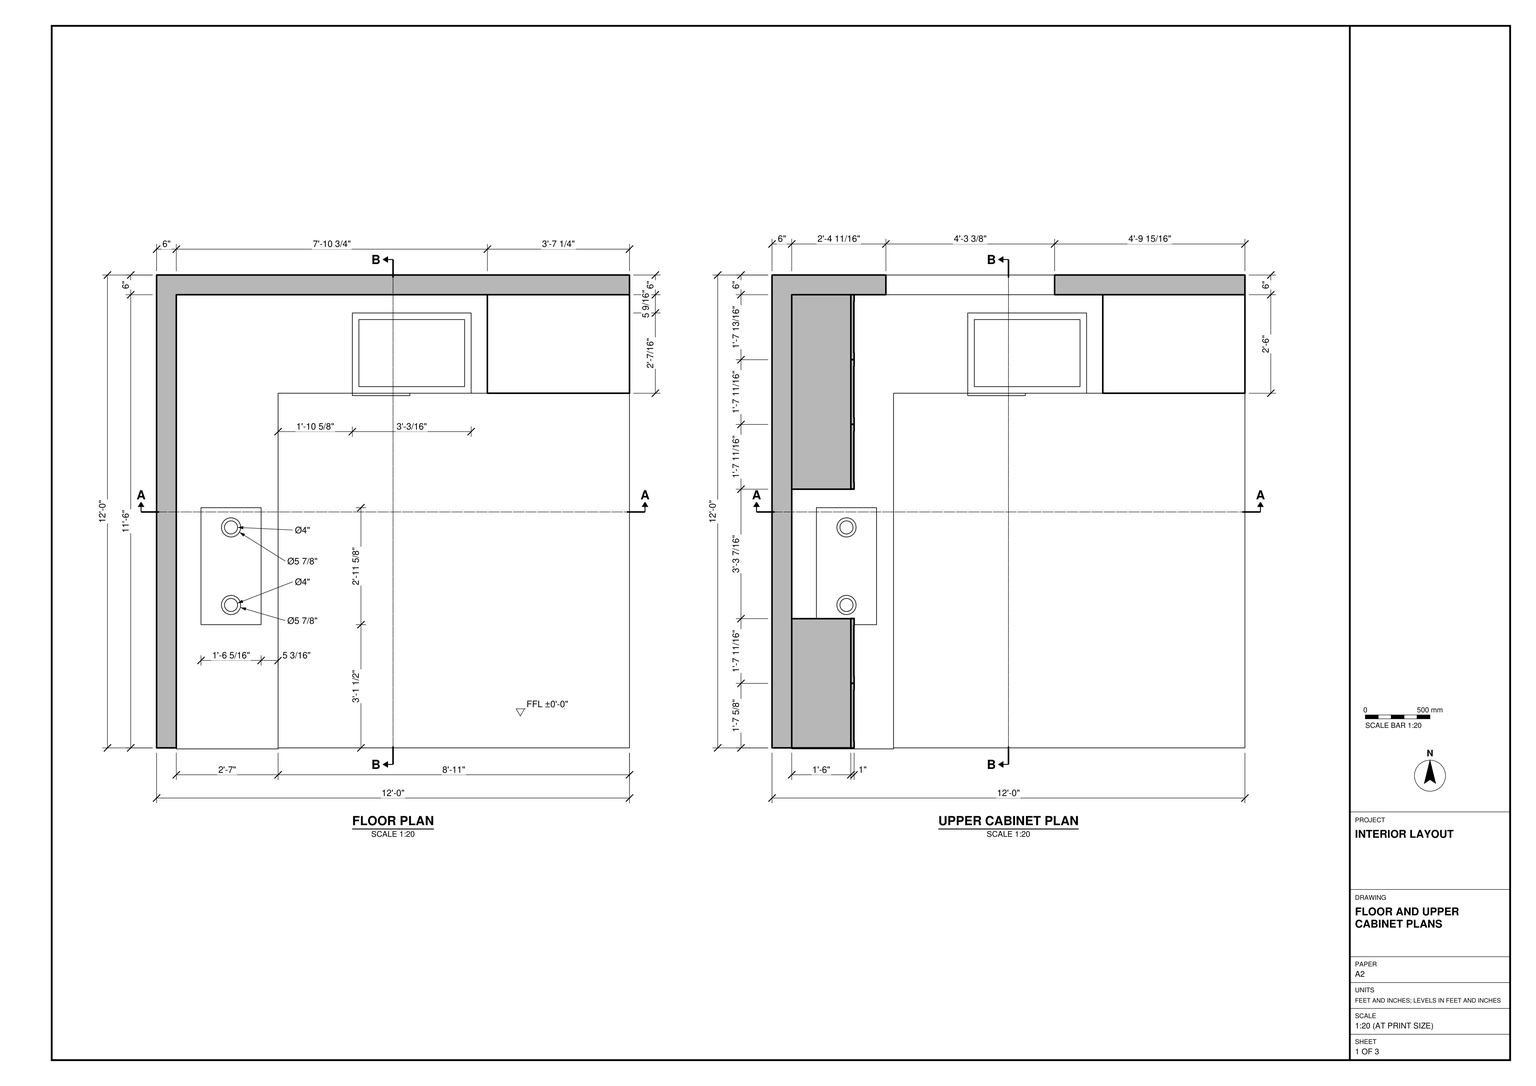
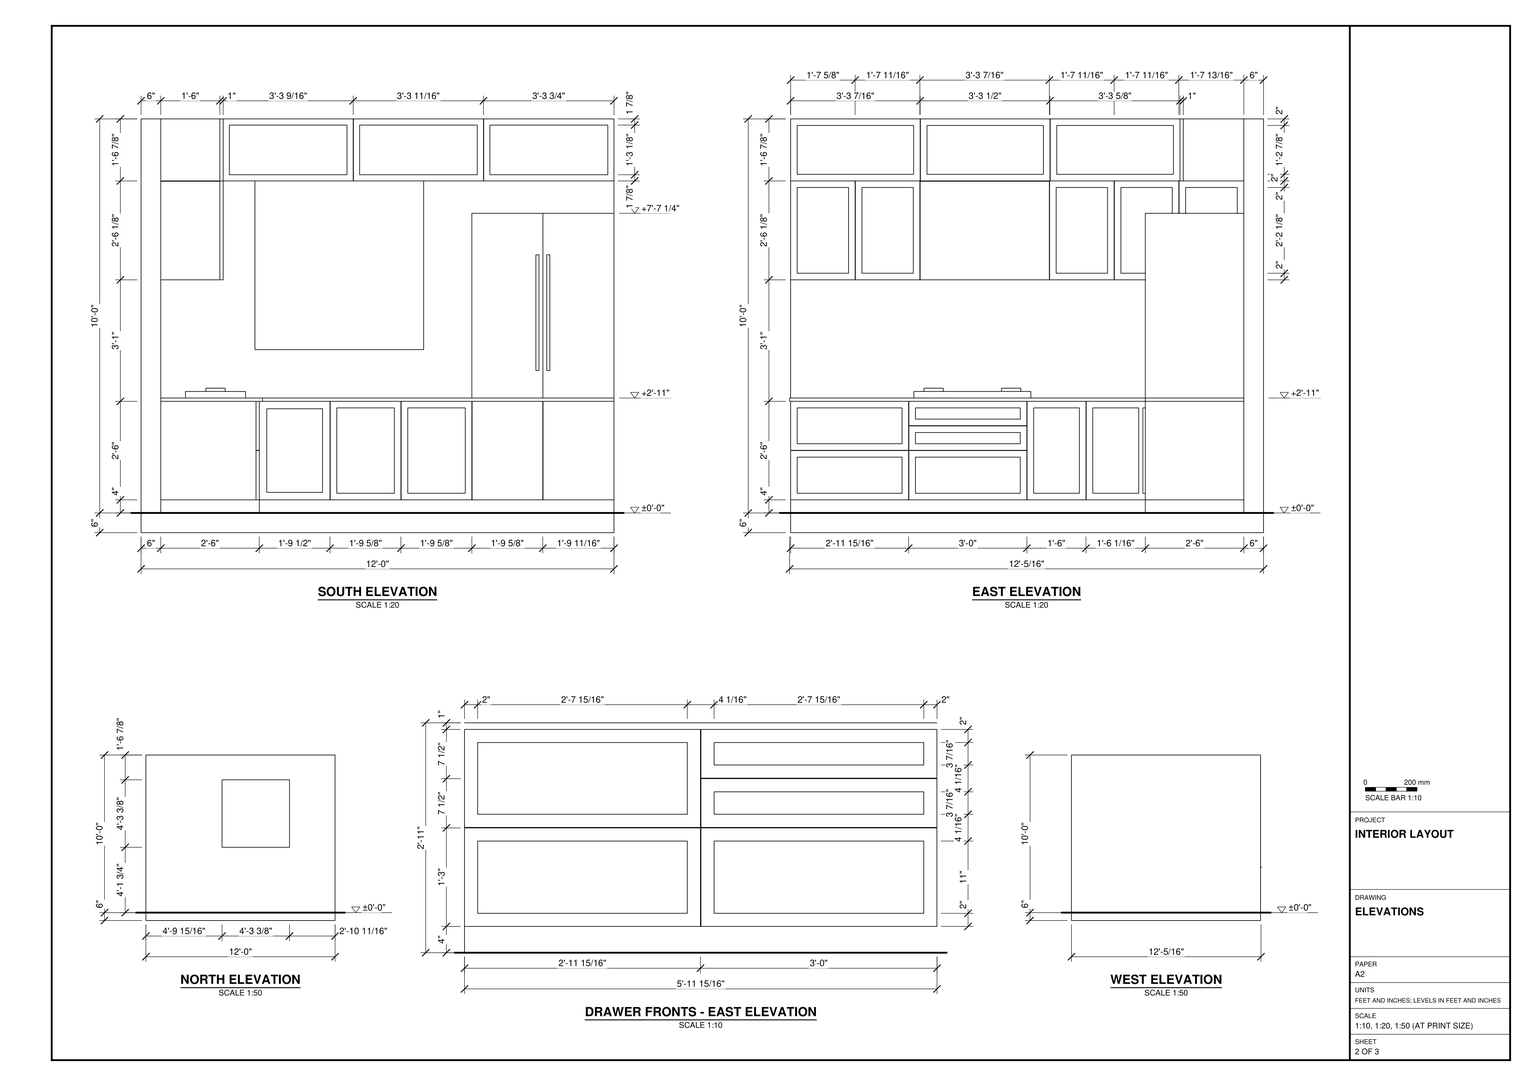
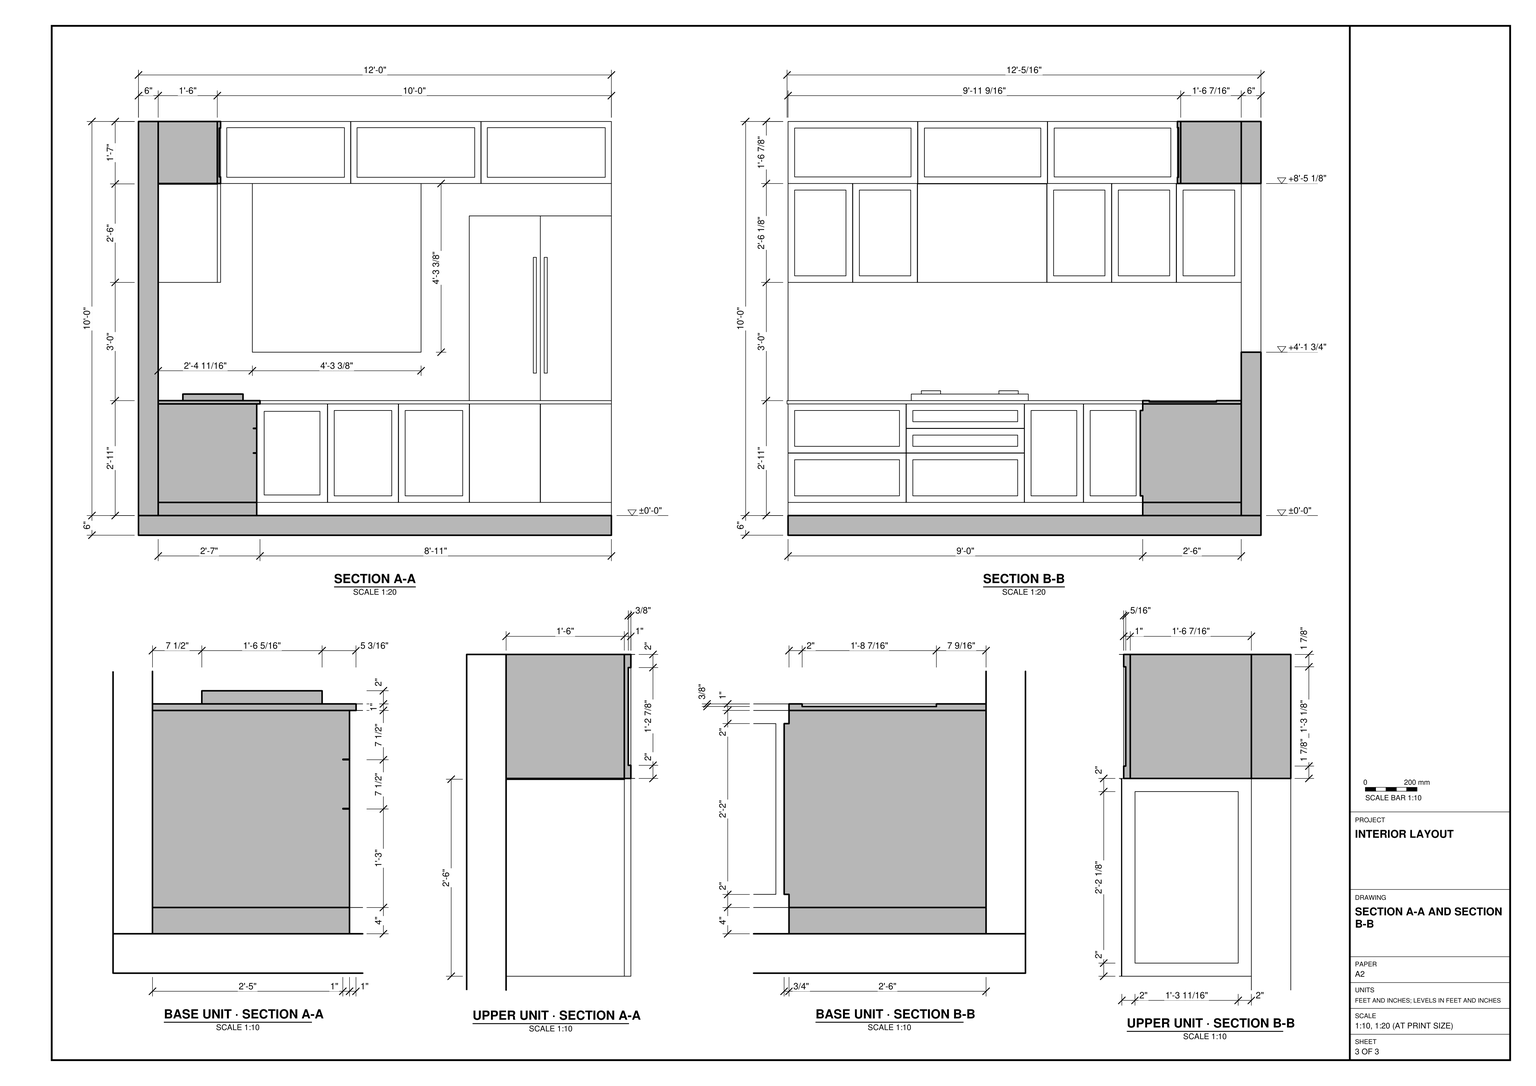
Use the plans, elevations, sections and joinery details in task_files/diagram_01.pdf to build the kitchen in SketchUp. Work in feet and inches. The overall model extents are 12'-0" along x, 12'-5/16" along y and 10'-6" along z. Set the single finished floor level at ±0'-0". Model the 6" floor slab and the two adjoining 6" walls, leaving the other sides open as drawn.

Fit the base cabinets and worktops around the inside corner. Place the cooktop on the run shown at the left of the floor plan and the rectangular sink beneath the window opening on the return. Place the tall double-fronted unit at the far end of the sink run. Use the east elevation and enlarged drawer detail to lay out the two adjacent drawer banks, distinguishing the shallow upper drawers from the deeper fronts below. Include the plinths, worktop overhangs and framed cabinet fronts shown in section and elevation. Follow the upper cabinet plan for the projecting wall units, keeping the space above the cooktop open below the top row.

Keep the walls, slab and each piece of joinery or furniture in separate groups or components, and use components for repeated parts. Decor and loose items, including appliances, may be any suitable library components. Save one SketchUp model as output_files/l_shaped_kitchen_with_fitted_cabinetry.skp.

# SketchUp Ruby script. Lengths in inches.
U = 1.inch
M = Sketchup.active_model
def pt(a) = Geom::Point3d.new(a.map { |v| v * U })
def face(e, loops, mat)
  f = e.add_face(loops[0].map { |a| pt(a) })
  loops[1..].each { |l| e.add_face(l.map { |a| pt(a) }).erase! }
  f.material = f.back_material = mat if mat
  f
end
# faces: each face lists its corners as indices into pts; further lists are holes
def faces(e, pts, list, mat = nil) = list.each { |f| face(e, (f[0].is_a?(Array) ? f : [f]).map { |l| l.map { |i| pts[i] } }, mat) }
# xy, xz, yz: faces in a plane at the given z, y or x. An outline is a flat list of corners, or four numbers for a rectangle; further outlines are holes
def ring(l) = l.size == 4 ? [[l[0], l[1]], [l[2], l[1]], [l[2], l[3]], [l[0], l[3]]] : l.each_slice(2).to_a
def flat(e, list, mat, &to3) = list.each { |f| face(e, (f[0].is_a?(Array) ? f : [f]).map { |l| ring(l).map { |u, v| to3.(u, v) } }, mat) }
def xy(e, z, list, mat = nil) = flat(e, list, mat) { |x, y| [x, y, z] }
def xz(e, y, list, mat = nil) = flat(e, list, mat) { |x, z| [x, y, z] }
def yz(e, x, list, mat = nil) = flat(e, list, mat) { |y, z| [x, y, z] }
def lines(e, pts, list) = list.each { |a, b| e.add_line(pt(pts[a]), pt(pts[b])) }
# prism: a flat outline (further loops are holes) pulled along v
def prism(e, loops, v, mat = nil)
  f = face(e, loops, mat); d = Geom::Vector3d.new(v.map { |x| x * U })
  f.pushpull(f.normal.samedirection?(d) ? d.length : -d.length)
end
def box(e, o, s, mat = nil) = prism(e, [[o, [o[0] + s[0], o[1], o[2]], [o[0] + s[0], o[1] + s[1], o[2]], [o[0], o[1] + s[1], o[2]]]], [0, 0, s[2]], mat)
def at(x, y, z, deg = 0) = Geom::Transformation.translation(pt([x, y, z])) * Geom::Transformation.rotation(ORIGIN, Z_AXIS, deg.degrees)
def axes(o, x, y, z) = Geom::Transformation.new([*x, 0, *y, 0, *z, 0, *pt(o).to_a, 1])
def part(name) = M.definitions.add(name)
# library, detail: a bought-in or finely detailed component or shape, given as its bounding box
def library(name, o, s) = part(name).tap { |d| box(d.entities, o, s) }
def detail(e, o, s) = box(e.add_group.entities, o, s)
def put(e, d, t, mat = nil) = e.add_instance(d, t).tap { |i| i.material = mat if mat }
def group(e, t, mat = nil) = e.add_group.tap { |g| g.transformation = t; g.material = mat if mat }.entities
root = M.entities
M.materials.add("[Aluminum]").color = [179, 179, 179]
M.materials.add("[Carrera Marble]").color = [207, 207, 207]
M.materials.add("[Granite Dark Gray]").color = [69, 68, 68]
M.materials.add("[Stone Vein Gray]").color = [166, 165, 165]
M.materials.add("[Terrazzo Light Blue]").color = [196, 214, 227]
M.materials.add("[Translucent Glass Sky Reflection]").color = [126, 138, 183]
M.materials["[Translucent Glass Sky Reflection]"].alpha = 0.52
M.materials.add("[White Subway Tile]").color = [243, 252, 253]
xy(root,35,[[13.51,37.83,31.83,73.46]])
xy(root,35,[[100.72,108.3125,144,138.3125]],"[Terrazzo Light Blue]")
xy(root,37,[[22.67,41.83,23.1875,41.9,23.67,42.1,24.08,42.42,24.4,42.83,24.6,43.32,24.67,43.83,24.6,44.35,24.4,44.83,24.08,45.25,23.67,45.57,23.1875,45.77,22.67,45.83,22.15,45.77,21.67,45.57,21.26,45.25,20.9375,44.83,20.74,44.35,20.67,43.83,20.74,43.32,20.9375,42.83,21.26,42.42,21.67,42.1,22.15,41.9]])
xy(root,37,[[[13.51,37.83,31.83,73.46],[22.67,40.9,21.91,41,21.2,41.29,20.59,41.76,20.125,42.37,19.83,43.07,19.73,43.83,19.83,44.59,20.125,45.3,20.59,45.91,21.2,46.38,21.91,46.67,22.67,46.77,23.43,46.67,24.14,46.38,24.75,45.91,25.21,45.3,25.51,44.59,25.61,43.83,25.51,43.07,25.21,42.37,24.75,41.76,24.14,41.29,23.43,41],[22.67,64.52,21.91,64.62,21.2,64.92,20.59,65.38,20.125,65.99,19.83,66.7,19.73,67.46,19.83,68.22,20.125,68.93,20.59,69.54,21.2,70,21.91,70.3,22.67,70.4,23.43,70.3,24.14,70,24.75,69.54,25.21,68.93,25.51,68.22,25.61,67.46,25.51,66.7,25.21,65.99,24.75,65.38,24.14,64.92,23.43,64.62]]],"[Stone Vein Gray]")
xy(root,38,[[[22.67,40.9,23.43,41,24.14,41.29,24.75,41.76,25.21,42.37,25.51,43.07,25.61,43.83,25.51,44.59,25.21,45.3,24.75,45.91,24.14,46.38,23.43,46.67,22.67,46.77,21.91,46.67,21.2,46.38,20.59,45.91,20.125,45.3,19.83,44.59,19.73,43.83,19.83,43.07,20.125,42.37,20.59,41.76,21.2,41.29,21.91,41],[22.67,41.83,22.15,41.9,21.67,42.1,21.26,42.42,20.9375,42.83,20.74,43.32,20.67,43.83,20.74,44.35,20.9375,44.83,21.26,45.25,21.67,45.57,22.15,45.77,22.67,45.83,23.1875,45.77,23.67,45.57,24.08,45.25,24.4,44.83,24.6,44.35,24.67,43.83,24.6,43.32,24.4,42.83,24.08,42.42,23.67,42.1,23.1875,41.9]],[[22.67,64.52,23.43,64.62,24.14,64.92,24.75,65.38,25.21,65.99,25.51,66.7,25.61,67.46,25.51,68.22,25.21,68.93,24.75,69.54,24.14,70,23.43,70.3,22.67,70.4,21.91,70.3,21.2,70,20.59,69.54,20.125,68.93,19.83,68.22,19.73,67.46,19.83,66.7,20.125,65.99,20.59,65.38,21.2,64.92,21.91,64.62],[22.67,65.46,22.15,65.53,21.67,65.73,21.26,66.05,20.9375,66.46,20.74,66.94,20.67,67.46,20.74,67.98,20.9375,68.46,21.26,68.875,21.67,69.19,22.15,69.39,22.67,69.46,23.1875,69.39,23.67,69.19,24.08,68.875,24.4,68.46,24.6,67.98,24.67,67.46,24.6,66.94,24.4,66.46,24.08,66.05,23.67,65.73,23.1875,65.53]]],"[Stone Vein Gray]")
xy(root,91.25,[[100.72,108.3125,144,138.3125]],"[Aluminum]")
xz(root,37.83,[[13.51,35,31.83,37]],"[Stone Vein Gray]")
xz(root,73.46,[[13.51,35,31.83,37]])
xz(root,108.3125,[[[100.72,35,122.36,91.25],[120.23,43.38,121.16,78.63]],[[122.36,35,144,91.25],[123.54,43.38,124.48,78.63]]],"[Aluminum]")
xz(root,108.3125,[[120.23,43.38,121.16,78.63],[123.54,43.38,124.48,78.63]],"[Terrazzo Light Blue]")
xz(root,138.3125,[[100.72,35,144,91.25]],"[Terrazzo Light Blue]")
yz(root,13.51,[[37.83,35,73.46,37]])
yz(root,31.83,[[37.83,35,73.46,37]],"[Stone Vein Gray]")
yz(root,100.72,[[108.3125,35,138.3125,91.25]],"[Aluminum]")
yz(root,144,[[108.3125,35,138.3125,91.25]],"[Aluminum]")
p = [[21.91,41,37],[22.67,40.9,37],[22.67,40.9,38],[21.91,41,38],[23.43,41,37],[23.43,41,38],
  [21.2,41.29,37],[21.2,41.29,38],[24.14,41.29,37],[24.14,41.29,38],[20.59,41.76,37],[20.59,41.76,38],
  [24.75,41.76,37],[24.75,41.76,38],[20.125,42.37,37],[20.125,42.37,38],[22.67,41.83,37],[22.15,41.9,37],
  [22.15,41.9,38],[22.67,41.83,38],[23.1875,41.9,37],[23.1875,41.9,38],[25.21,42.37,37],[25.21,42.37,38],
  [21.67,42.1,37],[21.67,42.1,38],[23.67,42.1,37],[23.67,42.1,38],[21.26,42.42,37],[21.26,42.42,38],
  [24.08,42.42,37],[24.08,42.42,38],[19.83,43.07,37],[19.83,43.07,38],[20.9375,42.83,37],[20.9375,42.83,38],
  [24.4,42.83,37],[24.4,42.83,38],[25.51,43.07,37],[25.51,43.07,38],[20.74,43.32,37],[20.74,43.32,38],
  [24.6,43.32,37],[24.6,43.32,38],[19.73,43.83,37],[19.73,43.83,38],[25.61,43.83,37],[25.61,43.83,38],
  [20.67,43.83,37],[20.67,43.83,38],[24.67,43.83,37],[24.67,43.83,38],[19.83,44.59,37],[19.83,44.59,38],
  [20.74,44.35,37],[20.74,44.35,38],[24.6,44.35,37],[24.6,44.35,38],[25.51,44.59,37],[25.51,44.59,38],
  [20.9375,44.83,37],[20.9375,44.83,38],[24.4,44.83,37],[24.4,44.83,38],[20.125,45.3,37],[20.125,45.3,38],
  [25.21,45.3,37],[25.21,45.3,38],[21.26,45.25,37],[21.26,45.25,38],[24.08,45.25,37],[24.08,45.25,38],
  [21.67,45.57,37],[21.67,45.57,38],[23.67,45.57,37],[23.67,45.57,38],[20.59,45.91,37],[20.59,45.91,38],
  [24.75,45.91,37],[24.75,45.91,38],[22.15,45.77,37],[22.15,45.77,38],[23.1875,45.77,37],[23.1875,45.77,38],
  [22.67,45.83,37],[22.67,45.83,38],[21.2,46.38,37],[21.2,46.38,38],[24.14,46.38,37],[24.14,46.38,38],
  [21.91,46.67,37],[21.91,46.67,38],[23.43,46.67,37],[23.43,46.67,38],[22.67,46.77,37],[22.67,46.77,38],
  [21.91,64.62,37],[22.67,64.52,37],[22.67,64.52,38],[21.91,64.62,38],[23.43,64.62,37],[23.43,64.62,38],
  [21.2,64.92,37],[21.2,64.92,38],[24.14,64.92,37],[24.14,64.92,38],[20.59,65.38,37],[20.59,65.38,38],
  [24.75,65.38,37],[24.75,65.38,38],[20.125,65.99,37],[20.125,65.99,38],[25.21,65.99,37],[25.21,65.99,38],
  [22.15,65.53,37],[21.67,65.73,37],[21.67,65.73,38],[22.15,65.53,38],[22.67,65.46,37],[22.67,65.46,38],
  [23.1875,65.53,37],[23.1875,65.53,38],[23.67,65.73,37],[23.67,65.73,38],[21.26,66.05,37],[21.26,66.05,38],
  [24.08,66.05,37],[24.08,66.05,38],[19.83,66.7,37],[19.83,66.7,38],[20.9375,66.46,37],[20.9375,66.46,38],
  [24.4,66.46,37],[24.4,66.46,38],[25.51,66.7,37],[25.51,66.7,38],[20.74,66.94,37],[20.74,66.94,38],
  [24.6,66.94,37],[24.6,66.94,38],[19.73,67.46,37],[19.73,67.46,38],[25.61,67.46,37],[25.61,67.46,38],
  [20.67,67.46,37],[20.67,67.46,38],[24.67,67.46,37],[24.67,67.46,38],[19.83,68.22,37],[19.83,68.22,38],
  [20.74,67.98,37],[20.74,67.98,38],[24.6,67.98,37],[24.6,67.98,38],[25.51,68.22,37],[25.51,68.22,38],
  [20.9375,68.46,37],[20.9375,68.46,38],[24.4,68.46,37],[24.4,68.46,38],[20.125,68.93,37],[20.125,68.93,38],
  [25.21,68.93,37],[25.21,68.93,38],[21.26,68.875,37],[21.26,68.875,38],[24.08,68.875,37],[24.08,68.875,38],
  [20.59,69.54,37],[20.59,69.54,38],[21.67,69.19,37],[21.67,69.19,38],[23.67,69.19,37],[23.67,69.19,38],
  [24.75,69.54,37],[24.75,69.54,38],[22.15,69.39,37],[22.15,69.39,38],[23.1875,69.39,37],[23.1875,69.39,38],
  [22.67,69.46,37],[22.67,69.46,38],[21.2,70,37],[21.2,70,38],[24.14,70,37],[24.14,70,38],
  [21.91,70.3,37],[21.91,70.3,38],[23.43,70.3,37],[23.43,70.3,38],[22.67,70.4,37],[22.67,70.4,38],
  [35,0.3125,34],[35,0.3125,19.08],[35,0.3125,4],[25,79.09,71],[25,79.09,101.12],[24,79.09,101.12],
  [24,79.09,71]]
faces(root,p,[[0,1,2,3],[1,4,5,2],[6,0,3,7],[4,8,9,5],[10,6,7,11],[8,12,13,9],[14,10,11,15],[12,22,23,13],
  [32,14,15,33],[22,38,39,23],[44,32,33,45],[38,46,47,39],[52,44,45,53],[46,58,59,47],[64,52,53,65],[58,66,67,59],
  [76,64,65,77],[66,78,79,67],[86,76,77,87],[78,88,89,79],[90,86,87,91],[88,92,93,89],[94,90,91,95],[92,94,95,93],
  [96,97,98,99],[97,100,101,98],[102,96,99,103],[100,104,105,101],[106,102,103,107],[104,108,109,105],[110,106,107,111],[108,112,113,109],
  [128,110,111,129],[112,134,135,113],[140,128,129,141],[134,142,143,135],[148,140,141,149],[142,154,155,143],[160,148,149,161],[154,162,163,155],
  [168,160,161,169],[162,174,175,163],[182,168,169,183],[174,184,185,175],[186,182,183,187],[184,188,189,185],[190,186,187,191],[188,190,191,189]],"[Stone Vein Gray]")
faces(root,p,[[16,17,18,19],[20,16,19,21],[17,24,25,18],[26,20,21,27],[24,28,29,25],[30,26,27,31],[28,34,35,29],[36,30,31,37],
  [34,40,41,35],[42,36,37,43],[40,48,49,41],[50,42,43,51],[48,54,55,49],[56,50,51,57],[54,60,61,55],[62,56,57,63],
  [60,68,69,61],[70,62,63,71],[68,72,73,69],[74,70,71,75],[72,80,81,73],[82,74,75,83],[80,84,85,81],[84,82,83,85],
  [114,115,116,117],[118,114,117,119],[120,118,119,121],[122,120,121,123],[115,124,125,116],[126,122,123,127],[124,130,131,125],[132,126,127,133],
  [130,136,137,131],[138,132,133,139],[136,144,145,137],[146,138,139,147],[144,150,151,145],[152,146,147,153],[150,156,157,151],[158,152,153,159],
  [156,164,165,157],[166,158,159,167],[164,170,171,165],[172,166,167,173],[170,176,177,171],[178,172,173,179],[176,180,181,177],[180,178,179,181]])
lines(root,p,[[192,193],[193,194],[195,196],[196,197],[198,195]])
g1 = group(root,at(0,0.3125,-6),"[Carrera Marble]")
box(g1,[0,0,0],[144,144,6])
g2 = group(root,at(0,0.3125,0),"[White Subway Tile]")
xy(g2,0,[[0,0,0,144,144,144,144,138,6,138,6,0]])
xy(g2,49.74,[[34.67,138,86.05,144]])
xy(g2,101.12,[[34.67,138,86.05,144]])
xy(g2,120,[[0,0,6,0,6,138,144,138,144,144,0,144]])
xz(g2,0,[[0,0,6,120]])
xz(g2,138,[[[6,0,144,120],[34.67,49.74,86.05,101.12]]],"[White Subway Tile]")
xz(g2,144,[[[0,0,144,120],[34.67,49.74,86.05,101.12]]])
yz(g2,0,[[0,0,144,120]])
yz(g2,6,[[0,0,138,120]],"[White Subway Tile]")
yz(g2,34.67,[[138,49.74,144,101.12]])
yz(g2,86.05,[[138,49.74,144,101.12]])
yz(g2,144,[[138,0,144,120]])
g3 = group(root,at(6,0.3125,0),"[Stone Vein Gray]")
xy(g3,0,[[0,0,30,138],[30,108,138,138]])
xy(g3,4,[[0,0,30,0,30,108,138,108,138,138,0,138]])
xz(g3,0,[[0,0,30,4]])
xz(g3,108,[[30,0,138,4]])
xz(g3,138,[[30,0,138,4]])
yz(g3,0,[[0,0,138,4]])
yz(g3,30,[[0,0,108,4]])
yz(g3,138,[[108,0,138,4]])
g4 = group(root,at(6,0.3125,4),"[Terrazzo Light Blue]")
xy(g4,0,[[0,0,0,138,30,138,30,90,29,90,29,89.921,30,89.921,30,36,29,36,29,35.921,30,35.921,30,0],[30,108,30,138,138,138,138,108,116.4,108,116.4,109,116.321,109,116.321,108,94.8,108,94.8,109,94.721,109,94.721,108,73.2,108,73.2,109,73.121,109,73.121,108,51.6,108,51.6,109,51.521,109,51.521,108]])
xy(g4,2,[[29.803,38,30,69.921],[29.803,74,30,87.921],[29.803,92,30,106],[53.6,107.259,71.121,108],[75.2,108,92.721,108.197]])
xy(g4,2.268,[[32.268,108,49.254,108.197]])
xy(g4,13,[[29.803,38,30,69.921]])
xy(g4,15,[[29,0,30,35.921],[29,36,30,71.921]])
xy(g4,15.079,[[29,0,30,35.921],[29,36,30,71.921]])
xy(g4,17.079,[[29.803,2,30,33.921],[29.882,38,30,69.921]])
xy(g4,20.5,[[29.882,38,30,69.921]])
xy(g4,22.5,[[29,36,30,71.921],[29,71.921,30,72]])
xy(g4,22.579,[[29,36,30,71.921]])
xy(g4,24.579,[[29.882,38,30,69.921]])
xy(g4,27.732,[[32.268,108,49.254,108.197]])
xy(g4,28,[[29.803,2,30,33.921],[29.882,38,30,69.921],[29.803,74,30,87.921],[29.803,92,30,106],[53.6,107.259,71.121,108],
  [75.2,108,92.721,108.197]])
xy(g4,30,[[0,0,30,0,30,35.921,29,35.921,29,36,30,36,30,71.921,29,71.921,29,72,30,72,30,89.921,29,89.921,29,90,30,90,30,108,51.521,108,51.521,109,51.6,109,51.6,108,73.121,108,73.121,109,73.2,109,73.2,108,94.721,108,94.721,109,94.8,109,94.8,108,116.321,108,116.321,109,116.4,109,116.4,108,138,108,138,138,0,138]])
xz(g4,0,[[0,0,30,0,30,15,29,15,29,15.079,30,15.079,30,30,0,30]])
xz(g4,2,[[29.803,17.079,30,28]])
xz(g4,33.921,[[29.803,17.079,30,22.5],[29.803,22.5,30,28]])
xz(g4,35.921,[[29,0,30,15],[29,15.079,30,22.5],[29,22.5,30,30]])
xz(g4,36,[[29,0,30,15],[29,15.079,30,22.5],[29,22.579,30,30]])
xz(g4,38,[[29.803,2,30,13],[29.882,17.079,30,20.5],[29.882,24.579,30,28]])
xz(g4,69.921,[[29.803,2,30,13],[29.882,17.079,30,20.5],[29.882,24.579,30,28]])
xz(g4,71.921,[[29,15,30,15.079],[29,22.579,30,30]])
xz(g4,72,[[29,22.5,30,30]])
xz(g4,74,[[29.803,2,30,15],[29.803,15,30,22.5],[29.803,22.5,30,28]])
xz(g4,87.921,[[29.803,2,30,28]])
xz(g4,89.921,[[29,0,30,30]])
xz(g4,90,[[29,0,30,30]])
xz(g4,92,[[29.803,2,30,28]])
xz(g4,106,[[29.803,2,30,28]])
xz(g4,107.259,[[53.6,2,71.121,28]])
xz(g4,108,[[[30,0,51.521,30],[32.268,2.268,49.254,27.732]],[[51.6,0,73.121,30],[53.6,2,71.121,28]],[[73.2,0,94.721,30],[75.2,2,92.721,28]]])
xz(g4,108,[[94.8,0,116.321,30],[116.4,0,138,30]],"[Aluminum]")
xz(g4,108.197,[[75.2,2,92.721,28],[32.268,2.268,49.254,27.732]])
xz(g4,109,[[51.521,0,51.6,30],[73.121,0,73.2,30],[94.721,0,94.8,30],[116.321,0,116.4,30]])
xz(g4,138,[[30,0,138,30]])
yz(g4,0,[[0,0,138,30]])
yz(g4,29,[[35.921,0,36,15],[89.921,0,90,30],[0,15,35.921,15.079],[36,15,71.921,15.079],[36,22.5,71.921,22.579],
  [71.921,22.5,72,30]])
yz(g4,29.803,[[38,2,69.921,13],[74,2,87.921,28],[92,2,106,28],[2,17.079,33.921,28]])
yz(g4,29.882,[[38,17.079,69.921,20.5],[38,24.579,69.921,28]])
yz(g4,30,[[[0,0,35.921,15],[2,2,33.921,13]],[[36,0,71.921,15],[38,2,69.921,13]],[71.921,0,72,15],[[72,0,89.921,30],[74,2,87.921,28]],[[90,0,108,30],[92,2,106,28]],
  [2,2,33.921,13],[71.921,15,72,22.5],[[0,15.079,35.921,30],[2,17.079,33.921,28]],[[36,15.079,71.921,22.5],[38,17.079,69.921,20.5]],[[36,22.579,71.921,30],[38,24.579,69.921,28]]])
yz(g4,32.268,[[108,2.268,108.197,27.732]])
yz(g4,49.254,[[108,2.268,108.197,27.732]])
yz(g4,51.521,[[108,0,109,30]])
yz(g4,51.6,[[108,0,109,30]])
yz(g4,53.6,[[107.259,2,108,28]])
yz(g4,71.121,[[107.259,2,108,28]])
yz(g4,73.121,[[108,0,109,30]])
yz(g4,73.2,[[108,0,109,30]])
yz(g4,75.2,[[108,2,108.197,28]])
yz(g4,92.721,[[108,2,108.197,28]])
yz(g4,94.721,[[108,0,109,30]])
yz(g4,94.8,[[108,0,109,30]])
yz(g4,116.321,[[108,0,109,30]])
yz(g4,116.4,[[108,0,109,30]])
yz(g4,138,[[108,0,138,30]],"[Aluminum]")
p = [[30,-0.001,15.079],[30,0,15.079],[30,36,15.079],[30,35.999,15.079],[30,36,22.579],[30,35.999,22.579]]
lines(g4,p,[[0,1],[2,3],[4,5]])
g5 = group(root,at(6,0.3125,34),"[Granite Dark Gray]")
xy(g5,0,[[0,-0.3125,0,138,138,138,138,108,31,108,31,-0.3125]])
xy(g5,0.61,[[55.6,110,87.79,130.4375]],"[Carrera Marble]")
xy(g5,1,[[0,-0.3125,31,-0.3125,31,108,53.6,108,53.6,132.4375,89.79,132.4375,89.79,108,138,108,138,138,0,138],[[53.6,108,89.79,132.4375],[55.6,110,87.79,130.4375]]])
xz(g5,-0.3125,[[0,0,31,1]])
xz(g5,108,[[31,0,138,1]])
xz(g5,110,[[55.6,0.61,87.79,1]])
xz(g5,130.4375,[[55.6,0.61,87.79,1]])
xz(g5,138,[[0,0,138,1]])
yz(g5,0,[[-0.3125,0,138,1]])
yz(g5,31,[[-0.3125,0,108,1]])
yz(g5,55.6,[[110,0.61,130.4375,1]])
yz(g5,87.79,[[110,0.61,130.4375,1]])
yz(g5,138,[[108,0,138,1]])
g6 = group(root,at(6,0.3125,71),"[Terrazzo Light Blue]")
xy(g6,0,[[18,0,19,19.64],[18,19.71,19,39.35],[18,78.86,19,98.49],[18,98.57,19,118.21],[18,118.29,19,138]])
xy(g6,2,[[18.92,2,19,17.64],[18.92,21.71,19,37.35],[18.92,80.86,19,96.49],[18.92,100.57,19,116.21],[18.92,120.29,19,136]])
xy(g6,28.12,[[18.92,2,19,17.64],[18.92,21.71,19,37.35],[18.92,80.86,19,96.49],[18.92,100.57,19,116.21],[18.92,120.29,19,136]])
xy(g6,30,[[0,39.35,18,78.78]])
xy(g6,30.12,[[18,0,19,19.64],[18,19.71,19,39.35],[18,78.86,19,98.49],[18,98.57,19,118.21],[18,118.29,19,138]])
xz(g6,0,[[18,0,19,30.12]])
xz(g6,2,[[18.92,2,19,28.12]])
xz(g6,17.64,[[18.92,2,19,28.12]])
xz(g6,19.64,[[18,0,19,30.12]])
xz(g6,19.71,[[18,0,19,30.12]])
xz(g6,21.71,[[18.92,2,19,28.12]])
xz(g6,37.35,[[18.92,2,19,28.12]])
xz(g6,39.35,[[18,0,19,30.12]])
xz(g6,39.43,[[18,0,19,30.12]])
xz(g6,78.78,[[18,0,19,30.12]])
xz(g6,78.86,[[18,0,19,30.12]])
xz(g6,80.86,[[18.92,2,19,28.12]])
xz(g6,96.49,[[18.92,2,19,28.12]])
xz(g6,98.49,[[18,0,19,30.12]])
xz(g6,98.57,[[18,0,19,30.12]])
xz(g6,100.57,[[18.92,2,19,28.12]])
xz(g6,116.21,[[18.92,2,19,28.12]])
xz(g6,118.21,[[18,0,19,30.12]])
xz(g6,118.29,[[18,0,19,30.12]])
xz(g6,120.29,[[18.92,2,19,28.12]])
xz(g6,136,[[18.92,2,19,28.12]])
xz(g6,138,[[18,0,19,30.12]])
yz(g6,18,[[0,0,19.64,30.12],[19.64,0,19.71,30.12],[19.71,0,39.35,30.12],[39.35,0,39.43,30],[78.78,0,78.86,30.12],
  [78.86,0,98.49,30.12],[98.49,0,98.57,30.12],[98.57,0,118.21,30.12],[118.21,0,118.29,30.12],[118.29,0,138,30.12],
  [39.35,30,39.43,30.12]])
yz(g6,18.92,[[2,2,17.64,28.12],[21.71,2,37.35,28.12],[80.86,2,96.49,28.12],[100.57,2,116.21,28.12],[120.29,2,136,28.12]],"[Translucent Glass Sky Reflection]")
yz(g6,19,[[[0,0,19.64,30.12],[2,2,17.64,28.12]],[[19.71,0,39.35,30.12],[21.71,2,37.35,28.12]],[[78.86,0,98.49,30.12],[80.86,2,96.49,28.12]],[[98.57,0,118.21,30.12],[100.57,2,116.21,28.12]],[[118.29,0,138,30.12],[120.29,2,136,28.12]]])
p = [[18,39.35,0],[0,39.35,0],[18,78.86,0],[0,78.86,0]]
lines(g6,p,[[0,1],[2,3]])
g7 = group(g6,at(0,0,0))
xz(g7,39.35,[[0,0,18,30]])
xz(g7,78.78,[[0,0,18,30]])
p = [[18,39.35,30],[18,39.35,30.12]]
lines(g7,p,[[0,1]])
g8 = group(g7,at(0,0,0))
xy(g8,0,[[0,0,18,39.35],[0,78.86,18,138]])
xy(g8,30,[[0,0,18,138]])
xz(g8,0,[[0,0,18,30]])
xz(g8,138,[[0,0,18,30]])
yz(g8,0,[[120,0,138,30]])
yz(g8,18,[[0,0,39.35,30],[78.78,0,138,30]])
p = [[0,39.35,0],[0,78.86,0],[18,78.78,30],[18,78.78,30.12],[18,39.35,30],[18,39.35,30.12]]
lines(g8,p,[[0,1],[2,3],[4,5]])
g9 = group(root,at(6,0.3125,101.12),"[Terrazzo Light Blue]")
xy(g9,0,[[0,0,18,119.5625],[0,119.5625,138,138]])
xy(g9,18.88,[[0,0,18,0,18,119.5625,138,119.5625,138,138,0,138]])
xz(g9,0,[[0,0,18,18.88]])
xz(g9,119.5625,[[18,0,138,18.88]])
xz(g9,138,[[0,0,138,18.88]])
yz(g9,18,[[0,0,119.5625,18.88]])
yz(g9,138,[[119.5625,0,138,18.88]])
g10 = group(root,at(24,0.3125,101.12),"[Terrazzo Light Blue]")
xy(g10,0,[[0,0,1,39.44],[0,39.52,1,78.96],[0,79.04,1,118.5625],[0,118.5625,40.59,119.5625],[40.67,118.5625,80.25,119.5625],
  [80.33,118.5625,120,119.5625]])
xy(g10,1.88,[[2.88,118.5625,38.71,118.875],[42.55,118.5625,78.375,118.875],[82.21,118.5625,118.12,118.875]])
xy(g10,2,[[0.61,2,1,37.44],[0.61,41.52,1,76.96],[0.6875,81.04,1,116.5625]])
xy(g10,16.88,[[0.61,2,1,37.44],[0.61,41.52,1,76.96],[0.6875,81.04,1,116.5625]])
xy(g10,17,[[2.88,118.5625,38.71,118.875],[42.55,118.5625,78.375,118.875],[82.21,118.5625,118.12,118.875]])
xy(g10,18.88,[[0,0,1,39.44],[0,39.52,1,78.96],[0,79.04,1,118.5625],[0,118.5625,40.59,119.5625],[40.67,118.5625,80.25,119.5625],
  [80.33,118.5625,120,119.5625]])
xz(g10,0,[[0,0,1,18.88]])
xz(g10,2,[[0.61,2,1,16.88]])
xz(g10,37.44,[[0.61,2,1,16.88]])
xz(g10,39.44,[[0,0,1,18.88]])
xz(g10,39.52,[[0,0,0.92,18.88],[0.92,0,1,18.88]])
xz(g10,41.52,[[0.61,2,1,16.88]])
xz(g10,76.96,[[0.61,2,1,16.88]])
xz(g10,78.96,[[0,0,1,18.88]])
xz(g10,79.04,[[0,0,0.92,18.88],[0.92,0,1,18.88]])
xz(g10,81.04,[[0.6875,2,1,16.88]])
xz(g10,116.5625,[[0.6875,2,1,16.88]])
xz(g10,118.5625,[[[1,0,40.59,18.88],[2.88,1.88,38.71,17]],[[40.67,0,80.25,18.88],[42.55,1.88,78.375,17]],[[80.33,0,120,18.88],[82.21,1.88,118.12,17]]])
xz(g10,118.875,[[2.88,1.88,38.71,17],[42.55,1.88,78.375,17],[82.21,1.88,118.12,17]])
xz(g10,119.5625,[[0,0,40.59,18.88],[40.59,0,40.67,18.88],[40.67,0,80.25,18.88],[80.25,0,80.33,18.88],[80.33,0,120,18.88]])
yz(g10,0,[[0,0,39.44,18.88],[39.44,0,39.52,18.88],[39.52,0,78.96,18.88],[78.96,0,79.04,18.88],[79.04,0,118.5625,18.88]])
yz(g10,0.61,[[2,2,37.44,16.88],[41.52,2,76.96,16.88]])
yz(g10,0.6875,[[81.04,2,116.5625,16.88]])
yz(g10,1,[[[0,0,39.44,18.88],[2,2,37.44,16.88]],[[39.52,0,78.96,18.88],[41.52,2,76.96,16.88]],[[79.04,0,118.5625,18.88],[81.04,2,116.5625,16.88]]])
yz(g10,2.88,[[118.5625,1.88,118.875,17]])
yz(g10,38.71,[[118.5625,1.88,118.875,17]])
yz(g10,40.59,[[118.5625,0,119.5625,18.88]])
yz(g10,40.67,[[118.5625,0,119.5625,18.88]])
yz(g10,42.55,[[118.5625,1.88,118.875,17]])
yz(g10,78.375,[[118.5625,1.88,118.875,17]])
yz(g10,80.25,[[118.5625,0,119.5625,18.88]])
yz(g10,80.33,[[118.5625,0,119.5625,18.88]])
yz(g10,82.21,[[118.5625,1.88,118.875,17]])
yz(g10,118.12,[[118.5625,1.88,118.875,17]])
yz(g10,120,[[118.5625,0,119.5625,18.88]])
